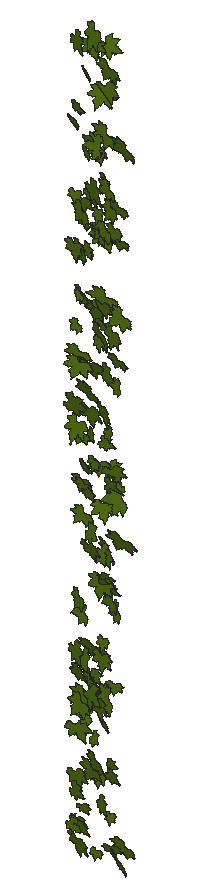
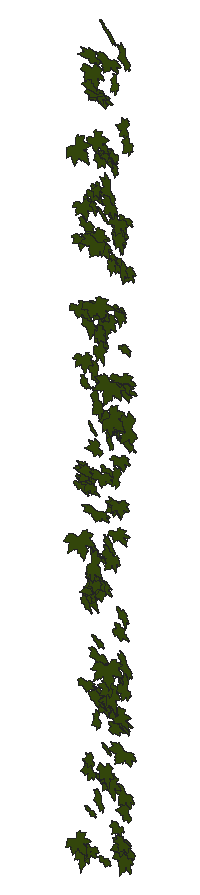
# SketchUp Ruby script. Lengths in inches.
U = 1.inch
M = Sketchup.active_model
def pt(a) = Geom::Point3d.new(a.map { |v| v * U })
def face(e, loops, mat)
  f = e.add_face(loops[0].map { |a| pt(a) })
  loops[1..].each { |l| e.add_face(l.map { |a| pt(a) }).erase! }
  f.material = f.back_material = mat if mat
  f
end
# faces: each face lists its corners as indices into pts; further lists are holes
def faces(e, pts, list, mat = nil) = list.each { |f| face(e, (f[0].is_a?(Array) ? f : [f]).map { |l| l.map { |i| pts[i] } }, mat) }
# xy, xz, yz: faces in a plane at the given z, y or x. An outline is a flat list of corners, or four numbers for a rectangle; further outlines are holes
def ring(l) = l.size == 4 ? [[l[0], l[1]], [l[2], l[1]], [l[2], l[3]], [l[0], l[3]]] : l.each_slice(2).to_a
def flat(e, list, mat, &to3) = list.each { |f| face(e, (f[0].is_a?(Array) ? f : [f]).map { |l| ring(l).map { |u, v| to3.(u, v) } }, mat) }
def xy(e, z, list, mat = nil) = flat(e, list, mat) { |x, y| [x, y, z] }
def xz(e, y, list, mat = nil) = flat(e, list, mat) { |x, z| [x, y, z] }
def yz(e, x, list, mat = nil) = flat(e, list, mat) { |y, z| [x, y, z] }
def lines(e, pts, list) = list.each { |a, b| e.add_line(pt(pts[a]), pt(pts[b])) }
# prism: a flat outline (further loops are holes) pulled along v
def prism(e, loops, v, mat = nil)
  f = face(e, loops, mat); d = Geom::Vector3d.new(v.map { |x| x * U })
  f.pushpull(f.normal.samedirection?(d) ? d.length : -d.length)
end
def box(e, o, s, mat = nil) = prism(e, [[o, [o[0] + s[0], o[1], o[2]], [o[0] + s[0], o[1] + s[1], o[2]], [o[0], o[1] + s[1], o[2]]]], [0, 0, s[2]], mat)
def at(x, y, z, deg = 0) = Geom::Transformation.translation(pt([x, y, z])) * Geom::Transformation.rotation(ORIGIN, Z_AXIS, deg.degrees)
def axes(o, x, y, z) = Geom::Transformation.new([*x, 0, *y, 0, *z, 0, *pt(o).to_a, 1])
def part(name) = M.definitions.add(name)
# library, detail: a bought-in or finely detailed component or shape, given as its bounding box
def library(name, o, s) = part(name).tap { |d| box(d.entities, o, s) }
def detail(e, o, s) = box(e.add_group.entities, o, s)
def put(e, d, t, mat = nil) = e.add_instance(d, t).tap { |i| i.material = mat if mat }
def group(e, t, mat = nil) = e.add_group.tap { |g| g.transformation = t; g.material = mat if mat }.entities
root = M.entities
M.materials.add("[Vegetation Blur 03]").color = [83, 114, 18]
c1 = part("ivy")
xy(c1.entities,0,[[0.782,0,0.786,0,0.787,0.005,0.789,0.009,0.821,0.072,0.875,0.147,1.001,0.272,1.073,0.331,1.137,0.363,1.178,0.379,1.223,0.384,1.272,0.383,1.311,0.374,1.36,0.355,1.399,0.334,1.491,0.285,1.541,0.244,1.583,0.199,1.617,0.15,1.64,0.128,1.662,0.115,1.717,0.105,1.745,0.093,1.784,0.054,1.819,0.057,1.854,0.064,1.882,0.075,1.896,0.074,1.91,0.071,1.937,0.063,1.964,0.053,1.99,0.038,2.016,0.015,2.034,0.002,2.04,0,2.038,0.003,2.036,0.007,2.033,0.038,2.036,0.068,2.045,0.1,2.055,0.116,2.064,0.123,2.077,0.129,2.088,0.129,2.106,0.132,2.118,0.13,2.179,0.132,2.207,0.133,2.225,0.133,2.242,0.138,2.22,0.162,2.207,0.186,2.206,0.213,2.212,0.236,2.228,0.262,2.247,0.274,2.298,0.283,2.355,0.294,2.37,0.296,2.376,0.295,2.377,0.3,2.377,0.303,2.385,0.329,2.411,0.37,2.426,0.392,2.449,0.407,2.511,0.426,2.561,0.444,2.619,0.466,2.589,0.469,2.561,0.476,2.501,0.5,2.449,0.516,2.424,0.523,2.401,0.535,2.377,0.556,2.372,0.568,2.36,0.575,2.268,0.586,2.225,0.592,2.207,0.599,2.194,0.61,2.143,0.65,2.13,0.664,2.122,0.682,2.123,0.7,2.13,0.719,2.148,0.75,2.17,0.781,2.195,0.807,2.221,0.828,2.284,0.874,2.291,0.88,2.288,0.887,2.276,0.9,2.267,0.916,2.265,0.933,2.273,0.967,2.292,1.002,2.313,1.03,2.334,1.054,2.348,1.067,2.358,1.074,2.363,1.076,2.362,1.081,2.35,1.094,2.347,1.11,2.35,1.143,2.359,1.18,2.385,1.254,2.415,1.324,2.448,1.393,2.45,1.4,2.446,1.398,2.44,1.394,2.427,1.383,2.402,1.36,2.376,1.339,2.345,1.324,2.305,1.309,2.282,1.303,2.273,1.306,2.245,1.294,2.212,1.287,2.187,1.291,2.163,1.301,2.142,1.316,2.134,1.327,2.124,1.325,2.09,1.292,2.053,1.259,2.014,1.234,1.973,1.215,1.954,1.21,1.931,1.208,1.909,1.212,1.893,1.22,1.879,1.233,1.872,1.248,1.867,1.281,1.864,1.319,1.821,1.258,1.773,1.197,1.726,1.141,1.698,1.121,1.679,1.116,1.666,1.117,1.647,1.122,1.632,1.129,1.62,1.141,1.617,1.154,1.617,1.219,1.621,1.254,1.623,1.268,1.623,1.281,1.618,1.314,1.606,1.346,1.603,1.375,1.607,1.403,1.603,1.467,1.599,1.499,1.605,1.525,1.614,1.552,1.629,1.577,1.635,1.589,1.629,1.587,1.618,1.582,1.596,1.566,1.581,1.556,1.568,1.552,1.557,1.55,1.545,1.553,1.531,1.562,1.522,1.572,1.504,1.591,1.486,1.611,1.474,1.631,1.457,1.666,1.455,1.684,1.457,1.698,1.452,1.715,1.444,1.728,1.424,1.754,1.419,1.772,1.423,1.786,1.434,1.819,1.444,1.848,1.446,1.855,1.44,1.861,1.43,1.867,1.386,1.904,1.349,1.948,1.326,1.973,1.31,1.995,1.288,2.048,1.284,2.153,1.287,2.254,1.284,2.255,1.282,2.253,1.278,2.247,1.274,2.237,1.266,2.216,1.226,2.125,1.208,2.076,1.184,2.033,1.155,1.984,1.135,1.942,1.111,1.899,1.083,1.861,1.053,1.85,1.059,1.83,1.061,1.809,1.056,1.79,1.049,1.767,1.04,1.749,1.018,1.733,0.994,1.726,0.942,1.734,0.95,1.6875,0.944,1.645,0.932,1.608,0.911,1.585,0.881,1.58,0.854,1.582,0.828,1.588,0.785,1.618,0.773,1.625,0.775,1.614,0.779,1.598,0.796,1.502,0.818,1.402,0.861,1.283,0.882,1.224,0.894,1.174,0.892,1.148,0.886,1.123,0.881,1.107,0.872,1.099,0.849,1.094,0.818,1.092,0.789,1.098,0.762,1.107,0.753,1.113,0.721,1.139,0.698,1.163,0.678,1.194,0.665,1.224,0.628,1.28,0.612,1.312,0.606,1.327,0.606,1.314,0.599,1.282,0.594,1.267,0.581,1.256,0.544,1.245,0.512,1.244,0.473,1.249,0.444,1.256,0.382,1.288,0.339,1.306,0.324,1.316,0.317,1.324,0.309,1.326,0.27,1.314,0.227,1.313,0.185,1.3125,0.152,1.317,0.122,1.328,0.092,1.345,0.073,1.353,0.079,1.338,0.092,1.308,0.117,1.249,0.13,1.215,0.139,1.164,0.147,1.148,0.157,1.136,0.163,1.122,0.174,1.086,0.177,1.067,0.182,1.054,0.186,1.043,0.191,1.038,0.211,1.028,0.237,1.005,0.25,0.974,0.253,0.96,0.25,0.944,0.242,0.914,0.243,0.906,0.249,0.902,0.26,0.894,0.289,0.88,0.307,0.873,0.322,0.862,0.364,0.799,0.403,0.738,0.431,0.709,0.439,0.691,0.441,0.678,0.4375,0.66,0.428,0.645,0.394,0.623,0.303,0.594,0.255,0.581,0.214,0.577,0.179,0.573,0.173,0.568,0.175,0.561,0.167,0.55,0.141,0.523,0.113,0.503,0.077,0.49,0.045,0.486,0.026,0.485,0.019,0.486,0.011,0.483,0,0.471,0.014,0.467,0.044,0.455,0.058,0.447,0.07,0.438,0.097,0.411,0.125,0.394,0.158,0.377,0.174,0.366,0.182,0.359,0.185,0.361,0.242,0.331,0.253,0.316,0.258,0.303,0.262,0.283,0.274,0.278,0.308,0.274,0.341,0.252,0.366,0.226,0.366,0.222,0.37,0.22,0.38,0.221,0.395,0.221,0.425,0.216,0.45,0.207,0.465,0.192,0.473,0.178,0.484,0.15,0.489,0.116,0.483,0.089,0.468,0.058,0.45,0.035,0.435,0.018,0.429,0.011,0.434,0.012,0.438,0.014,0.469,0.019,0.542,0.016,0.581,0.015,0.612,0.027,0.68,0.055,0.696,0.057,0.712,0.052,0.73,0.045,0.741,0.036,0.766,0.014]])
put(root,c1,axes([79.86,173.7,54.72],[0.18512,0.00647,0.33943],[0.41367,-0.0999,-0.14998],[-0.04308,-0.93144,0.01844]),"[Vegetation Blur 03]")
put(root,c1,axes([80.13,173.7,87.79],[0.32765,-0.02489,0.01881],[0.02157,-0.07508,-0.26601],[-0.01455,-0.67173,0.02903]),"[Vegetation Blur 03]")
put(root,c1,axes([80.16,173.7,79.85],[0.50815,0.02983,-0.17456],[-0.21367,-0.02159,-0.41487],[0.01743,-1.13431,0.00331]),"[Vegetation Blur 03]")
put(root,c1,axes([80.49,173.7,81.24],[0.24945,-0.08617,-0.15972],[-0.19859,-0.02674,-0.20432],[-0.02483,-0.6519,0.02949]),"[Vegetation Blur 03]")
put(root,c1,axes([80.01,173.7,91.5625],[0.34754,-0.2147,0.09746],[0.13272,0.06991,-0.29103],[-0.08677,-0.75297,-0.05481]),"[Vegetation Blur 03]")
put(root,c1,axes([81.18,173.7,78.04],[0.15268,0.21133,-0.48982],[-0.60568,0.18355,-0.11329],[-0.06257,-1.26109,-0.09857]),"[Vegetation Blur 03]")
put(root,c1,axes([80.14,173.7,79.3],[0.55742,0.02012,-0.13001],[-0.15728,-0.13301,-0.4524],[0.0271,-1.18554,0.04855]),"[Vegetation Blur 03]")
put(root,c1,axes([79.89,173.7,85.24],[0.58629,-0.17522,0.04019],[0.04988,0.00183,-0.48347],[-0.08478,-1.21072,-0.00655]),"[Vegetation Blur 03]")
put(root,c1,axes([80.37,173.7,75.5],[0.38921,0.02788,-0.11804],[-0.14492,0.01541,-0.31769],[0.01009,-0.85429,-0.00958]),"[Vegetation Blur 03]")
put(root,c1,axes([80.71,173.7,87.32],[0.36249,-0.1648,-0.3565],[-0.41016,0.32061,-0.3011],[-0.17026,-1.12322,-0.03364]),"[Vegetation Blur 03]")
put(root,c1,axes([80.36,173.7,73.16],[0.40951,0.01971,-0.10583],[-0.13003,0.06915,-0.33309],[-0.00105,-0.88123,-0.0285]),"[Vegetation Blur 03]")
put(root,c1,axes([80.13,173.7,55.37],[0.37849,-0.06704,0.09137],[0.11442,0.06293,-0.30843],[-0.02244,-0.80977,-0.03153]),"[Vegetation Blur 03]")
put(root,c1,axes([79.76,173.7,60.03],[0.53376,0.03726,0.21952],[0.269,0.00727,-0.43585],[0.01776,-1.22992,0.00407]),"[Vegetation Blur 03]")
put(root,c1,axes([80.72,173.7,62.45],[0.42826,-0.11256,-0.35023],[-0.42906,0.04831,-0.35189],[-0.05529,-1.24664,0.01798]),"[Vegetation Blur 03]")
put(root,c1,axes([79.82,173.7,76.28],[0.20202,-0.16973,0.51163],[0.63222,0.07532,-0.16235],[0.00985,-1.35325,-0.07321]),"[Vegetation Blur 03]")
put(root,c1,axes([81.05,173.7,66.72],[0.19822,-0.13225,-0.36337],[-0.44645,0.06503,-0.16594],[-0.0552,-1.0008,0.03723]),"[Vegetation Blur 03]")
put(root,c1,axes([80.13,173.7,56.5],[0.13655,-0.05783,0.35944],[0.43753,-0.10617,-0.1134],[-0.05764,-0.9429,-0.00928]),"[Vegetation Blur 03]")
put(root,c1,axes([80.49,173.7,62.03],[0.51915,-0.17766,-0.225],[-0.28069,-0.03421,-0.42714],[-0.06834,-1.20911,0.04515]),"[Vegetation Blur 03]")
put(root,c1,axes([79.91,173.7,57.74],[0.52125,-0.12471,0.19571],[0.23821,-0.0569,-0.42827],[-0.06661,-1.17932,-0.00003]),"[Vegetation Blur 03]")
put(root,c1,axes([80.65,173.7,71.69],[0.40363,-0.02669,-0.22372],[-0.27442,-0.04788,-0.32887],[0.00236,-1.00289,0.02165]),"[Vegetation Blur 03]")
put(root,c1,axes([80.59,173.7,73.06],[0.38167,-0.01698,-0.15187],[-0.18516,0.0606,-0.31101],[-0.02031,-0.87168,-0.01866]),"[Vegetation Blur 03]")
put(root,c1,axes([80.47,173.7,67.37],[0.45232,-0.27078,-0.13351],[-0.16346,0.04761,-0.38403],[-0.13176,-0.98864,0.01808]),"[Vegetation Blur 03]")
put(root,c1,axes([80.62,173.7,82.86],[0.28246,-0.12607,-0.06429],[-0.08477,-0.04633,-0.23378],[-0.05266,-0.60166,0.03147]),"[Vegetation Blur 03]")
put(root,c1,axes([80.58,173.7,87.18],[0.47471,-0.2198,-0.23723],[-0.27334,0.21714,-0.39597],[-0.14555,-1.12467,-0.03009]),"[Vegetation Blur 03]")
put(root,c1,axes([81.07,173.7,79.25],[0.13027,0.06294,-0.24641],[-0.30303,0.06322,-0.10416],[-0.01626,-0.67369,-0.0328]),"[Vegetation Blur 03]")
put(root,c1,axes([80.01,173.7,54.72],[0.66178,-0.29714,0.00728],[0.02239,0.12543,-0.55031],[-0.14293,-1.35615,-0.0525]),"[Vegetation Blur 03]")
put(root,c1,axes([80.57,173.7,87.5],[0.50423,-0.25138,-0.23976],[-0.28758,0.12452,-0.42338],[-0.1361,-1.1944,0.00632]),"[Vegetation Blur 03]")
put(root,c1,axes([80.39,173.7,91.92],[0.06833,-0.14193,0.31087],[0.38368,-0.0807,-0.06197],[-0.05132,-0.79223,-0.04938]),"[Vegetation Blur 03]")
put(root,c1,axes([80.48,173.7,85.44],[0.499,-0.30069,-0.16614],[-0.19194,0.14146,-0.42426],[-0.16109,-1.09995,-0.00914]),"[Vegetation Blur 03]")
put(root,c1,axes([80.16,173.7,76.24],[0.61381,-0.2023,0.00115],[-0.01893,-0.26118,-0.49641],[-0.09648,-1.23581,0.10472]),"[Vegetation Blur 03]")
put(root,c1,axes([80.52,173.7,83.02],[0.4623,-0.23108,-0.11744],[-0.13279,0.12742,-0.38762],[-0.12523,-0.98816,-0.02252]),"[Vegetation Blur 03]")
put(root,c1,axes([80.3,173.7,87.6],[0.49002,-0.06773,0.03255],[0.04203,0.06603,-0.39982],[-0.03013,-1.00954,-0.02833]),"[Vegetation Blur 03]")
put(root,c1,axes([80.17,173.7,62.87],[0.2552,-0.21443,0.36363],[0.45118,-0.05704,-0.2162],[-0.07626,-1.05507,-0.06222]),"[Vegetation Blur 03]")
put(root,c1,axes([80.04,173.7,64.1],[0.40591,-0.18014,0.3374],[0.39655,-0.24525,-0.33836],[-0.14603,-1.16675,0.01903]),"[Vegetation Blur 03]")
put(root,c1,axes([80.51,173.7,56.02],[0.2717,-0.01326,0.11926],[0.14597,0.06528,-0.22036],[0.00938,-0.63148,-0.02528]),"[Vegetation Blur 03]")
put(root,c1,axes([80.29,173.7,54.9],[0.29257,-0.13243,0.26003],[0.3239,0.04481,-0.23915],[-0.02726,-0.88901,-0.05079]),"[Vegetation Blur 03]")
put(root,c1,axes([80.16,173.7,95.55],[0.32606,-0.15993,0.37004],[0.43652,-0.25327,-0.27342],[-0.14515,-1.12098,0.00898]),"[Vegetation Blur 03]")
put(root,c1,axes([81.08,173.7,63.5625],[0.44681,-0.13861,-0.40686],[-0.47518,0.33403,-0.36549],[-0.1651,-1.33648,-0.04915]),"[Vegetation Blur 03]")
put(root,c1,axes([81.5,173.7,61.41],[0.05855,-0.11186,-0.32035],[-0.39567,-0.06136,-0.0448],[0.02177,-0.81436,0.04738]),"[Vegetation Blur 03]")
put(root,c1,axes([80.75,173.7,64.84],[0.5883,0.12569,-0.22776],[-0.28567,0.25569,-0.4693],[0.00068,-1.31528,-0.113]),"[Vegetation Blur 03]")
put(root,c1,axes([80.97,173.7,90.33],[0.2858,-0.16556,-0.09391],[-0.1058,0.0991,-0.24194],[-0.0923,-0.62621,-0.01346]),"[Vegetation Blur 03]")
put(root,c1,axes([80.41,173.7,79.23],[0.67545,-0.01499,0.0047],[0.00705,0.26519,-0.54115],[-0.00605,-1.36446,-0.10523]),"[Vegetation Blur 03]")
put(root,c1,axes([81.05,173.7,85.39],[0.30779,-0.16022,-0.12096],[-0.12595,0.19898,-0.2549],[-0.11031,-0.67423,-0.04648]),"[Vegetation Blur 03]")
put(root,c1,axes([80.5625,173.7,63.51],[0.22572,0.02556,0.3673],[0.42622,-0.34586,-0.17068],[-0.14503,-0.97663,0.07006]),"[Vegetation Blur 03]")
put(root,c1,axes([80.84,173.7,90.75],[0.27595,-0.07999,0.10883],[0.13684,0.05207,-0.2251],[-0.02378,-0.62852,-0.0325]),"[Vegetation Blur 03]")
put(root,c1,axes([81,173.7,58.78],[0.5571,-0.15804,-0.2532],[-0.30286,0.14883,-0.45846],[-0.10211,-1.30372,-0.02164]),"[Vegetation Blur 03]")
put(root,c1,axes([80.73,173.7,84.92],[0.26922,-0.1042,0.25304],[0.30661,-0.09593,-0.2235],[-0.06845,-0.83952,-0.00587]),"[Vegetation Blur 03]")
put(root,c1,axes([80.91,173.7,73.57],[0.07402,-0.1812,0.31745],[0.39109,-0.12634,-0.07209],[-0.07805,-0.80492,-0.06015]),"[Vegetation Blur 03]")
put(root,c1,axes([80.85,173.7,94.38],[0.3403,-0.29163,0.09942],[0.13762,0.03874,-0.29588],[-0.12643,-0.74278,-0.05447]),"[Vegetation Blur 03]")
put(root,c1,axes([80.82,173.7,72.4],[0.28875,-0.1223,0.18363],[0.229,0.01809,-0.23796],[-0.04139,-0.75306,-0.03554]),"[Vegetation Blur 03]")
put(root,c1,axes([80.6,173.7,76.96],[0.63148,-0.16792,0.0994],[0.12538,0.04433,-0.51879],[-0.07597,-1.32267,-0.03001]),"[Vegetation Blur 03]")
put(root,c1,axes([80.86,173.7,62.93],[0.31712,0.01449,0.22059],[0.2693,0.0595,-0.25849],[0.0241,-0.85537,-0.01424]),"[Vegetation Blur 03]")
put(root,c1,axes([80.71,173.7,95.6875],[0.52799,0.03971,0.1403],[0.17249,-0.03446,-0.43082],[0.01316,-1.14211,0.01788]),"[Vegetation Blur 03]")
put(root,c1,axes([81,173.7,82.47],[0.55471,-0.15442,-0.09413],[-0.10485,0.16405,-0.45388],[-0.08911,-1.1543,-0.05191]),"[Vegetation Blur 03]")
put(root,c1,axes([80.72,173.7,69.86],[0.52924,-0.21641,0.13482],[0.17446,0.07604,-0.43695],[-0.08896,-1.13835,-0.05482]),"[Vegetation Blur 03]")
put(root,c1,axes([81.3125,173.7,59.23],[0.48731,-0.17978,-0.24983],[-0.29064,0.21865,-0.40235],[-0.12987,-1.16387,-0.037]),"[Vegetation Blur 03]")
put(root,c1,axes([81.03,173.7,70.02],[0.07963,0.08394,0.36792],[0.43963,-0.2386,-0.05481],[-0.10777,-0.91131,0.04824]),"[Vegetation Blur 03]")
put(root,c1,axes([81.71,173.7,86.43],[0.27575,-0.07071,-0.32237],[-0.38727,0.16418,-0.22631],[-0.08498,-0.9776,-0.01469]),"[Vegetation Blur 03]")
put(root,c1,axes([81.58,173.7,90.93],[0.3287,-0.1611,-0.24597],[-0.30329,0.03864,-0.27395],[-0.07054,-0.91688,0.03167]),"[Vegetation Blur 03]")
put(root,c1,axes([80.88,173.7,87.98],[0.42324,-0.15513,0.17492],[0.21736,0.00516,-0.3496],[-0.06611,-0.97622,-0.02964]),"[Vegetation Blur 03]")
put(root,c1,axes([82.03,173.7,91.27],[0.20332,-0.17652,-0.4378],[-0.54125,0.03497,-0.16965],[-0.04646,-1.17997,0.06046]),"[Vegetation Blur 03]")
put(root,c1,axes([81.26,173.7,62.13],[0.08923,-0.0651,0.22881],[0.28147,0.0622,-0.07033],[0.01942,-0.60224,-0.032]),"[Vegetation Blur 03]")
put(root,c1,axes([81.3,173.7,74.42],[0.35274,-0.11868,-0.02991],[-0.03922,-0.02703,-0.29129],[-0.05595,-0.72928,0.01566]),"[Vegetation Blur 03]")
put(root,c1,axes([81.29,173.7,59.58],[0.08406,0.07505,0.23958],[0.28752,-0.16835,-0.0589],[-0.06954,-0.60538,0.04608]),"[Vegetation Blur 03]")
put(root,c1,axes([81.18,173.7,75.51],[0.18332,-0.13201,0.23981],[0.28131,-0.17522,-0.15841],[-0.10639,-0.6908,-0.00565]),"[Vegetation Blur 03]")
put(root,c1,axes([82.29,173.7,70.12],[0.10735,0.13666,-0.49936],[-0.59338,0.3622,-0.06937],[-0.16335,-1.22594,-0.07616]),"[Vegetation Blur 03]")
put(root,c1,axes([81.4,173.7,54.17],[0.29298,-0.03076,-0.00517],[-0.00747,-0.046,-0.2387],[-0.01442,-0.60127,0.01853]),"[Vegetation Blur 03]")
put(root,c1,axes([81.86,173.7,81.08],[0.29122,-0.09132,-0.34949],[-0.40801,0.28097,-0.238],[-0.13739,-1.02797,-0.034]),"[Vegetation Blur 03]")
put(root,c1,axes([82,173.7,81.86],[0.15958,-0.02123,-0.31626],[-0.37905,0.17205,-0.12921],[-0.08118,-0.84504,-0.01836]),"[Vegetation Blur 03]")
put(root,c1,axes([80.88,173.7,61.62],[0.16056,0.04012,0.53459],[0.63688,-0.33645,-0.12344],[-0.15436,-1.34643,0.04677]),"[Vegetation Blur 03]")
put(root,c1,axes([81.23,173.7,74.21],[0.45127,0.0715,0.00789],[0.01018,-0.0128,-0.36935],[0.0346,-0.92876,0.0057]),"[Vegetation Blur 03]")
put(root,c1,axes([81.72,173.7,83.38],[0.53259,0.07407,-0.33493],[-0.4092,-0.06459,-0.43565],[0.04766,-1.38209,0.00241]),"[Vegetation Blur 03]")
put(root,c1,axes([82.09,173.7,91.9375],[0.36403,-0.06267,-0.40957],[-0.5016,0.04126,-0.29795],[-0.03412,-1.27511,0.01049]),"[Vegetation Blur 03]")
put(root,c1,axes([82.07,173.7,89.21],[0.19632,-0.0358,-0.23719],[-0.2774,0.19596,-0.15758],[-0.08838,-0.69459,-0.03223]),"[Vegetation Blur 03]")
put(root,c1,axes([81.58,173.7,90.38],[0.31483,-0.06922,0.03461],[0.04453,0.03834,-0.25772],[-0.03078,-0.65259,-0.01881]),"[Vegetation Blur 03]")
put(root,c1,axes([81.85,173.7,86.875],[0.46325,-0.03451,-0.29794],[-0.36488,0.02419,-0.37832],[-0.02045,-1.21347,0.00093]),"[Vegetation Blur 03]")
put(root,c1,axes([81.33,173.7,97],[0.61554,-0.40401,-0.01131],[-0.04771,-0.21545,-0.519],[-0.19095,-1.24853,0.09322]),"[Vegetation Blur 03]")
put(root,c1,axes([81.55,173.7,81.5],[0.58606,-0.32249,-0.17371],[-0.19607,0.18401,-0.49434],[-0.17725,-1.2698,-0.02752]),"[Vegetation Blur 03]")
put(root,c1,axes([80.99,173.7,88.22],[0.41734,-0.25524,0.42347],[0.50918,-0.21404,-0.35453],[-0.15923,-1.35344,-0.02379]),"[Vegetation Blur 03]")
put(root,c1,axes([81.62,173.7,58.16],[0.34421,-0.10508,0.04416],[0.04441,-0.1326,-0.28022],[-0.05969,-0.70465,0.04615]),"[Vegetation Blur 03]")
put(root,c1,axes([81.58,173.7,87.36],[0.35292,-0.17211,0.08002],[0.07901,-0.17569,-0.29156],[-0.10181,-0.73298,0.0511]),"[Vegetation Blur 03]")
put(root,c1,axes([81.55,173.7,80.67],[0.3385,-0.12078,0.12895],[0.14584,-0.15588,-0.27795],[-0.08451,-0.75275,0.03687]),"[Vegetation Blur 03]")
put(root,c1,axes([81.34,173.7,68.47],[0.64834,-0.11558,0.00243],[-0.00125,-0.10055,-0.52962],[-0.05623,-1.33037,0.03982]),"[Vegetation Blur 03]")
put(root,c1,axes([82.33,173.7,89.03],[0.26205,-0.06963,-0.34462],[-0.42004,0.08964,-0.2156],[-0.05487,-1.01871,0.00458]),"[Vegetation Blur 03]")
put(root,c1,axes([81.55,173.7,93.82],[0.58164,-0.02914,-0.08506],[-0.10504,-0.22356,-0.46637],[0.00547,-1.19524,0.0893]),"[Vegetation Blur 03]")
put(root,c1,axes([82.47,173.7,63.02],[0.29249,-0.26424,-0.46367],[-0.56799,0.1604,-0.25303],[-0.12902,-1.30512,0.06278]),"[Vegetation Blur 03]")
put(root,c1,axes([81.86,173.7,68.43],[0.29824,-0.02143,-0.02343],[-0.02665,0.10046,-0.24043],[-0.01491,-0.60833,-0.03888]),"[Vegetation Blur 03]")
put(root,c1,axes([81.21,173.7,86.03],[0.60611,0.08882,0.16972],[0.20851,-0.00255,-0.49577],[0.04043,-1.31863,0.01239]),"[Vegetation Blur 03]")
put(root,c1,axes([81.375,173.7,72.07],[0.5345,0.11261,0.12686],[0.16236,-0.17388,-0.43135],[0.02823,-1.13219,0.07887]),"[Vegetation Blur 03]")
put(root,c1,axes([81.55,173.7,82.49],[0.44672,-0.11391,0.09884],[0.12385,0.0351,-0.3665],[-0.0489,-0.9518,-0.02535]),"[Vegetation Blur 03]")
put(root,c1,axes([81.8125,173.7,65.28],[0.33589,-0.10606,0.03492],[0.03467,-0.10992,-0.27466],[-0.05731,-0.68805,0.03849]),"[Vegetation Blur 03]")
put(root,c1,axes([81.28,173.7,62.03],[0.57796,-0.29472,0.19025],[0.2281,-0.10009,-0.48593],[-0.15109,-1.27852,-0.00582]),"[Vegetation Blur 03]")
put(root,c1,axes([81.71,173.7,90.2],[0.24496,-0.07431,0.21292],[0.23492,-0.26987,-0.19483],[-0.11909,-0.6852,0.05364]),"[Vegetation Blur 03]")
put(root,c1,axes([81.5,173.7,64.54],[0.56428,-0.16916,0.04285],[0.04868,-0.06133,-0.46503],[-0.08453,-1.16458,0.01826]),"[Vegetation Blur 03]")
put(root,c1,axes([81.55,173.7,69.47],[0.29882,0.02623,0.28715],[0.33985,-0.26962,-0.23169],[-0.09199,-0.91085,0.07685]),"[Vegetation Blur 03]")
put(root,c1,axes([81.77,173.7,74.99],[0.12471,-0.00455,0.29508],[0.36083,0.05141,-0.10146],[0.0229,-0.78534,-0.00835]),"[Vegetation Blur 03]")
put(root,c1,axes([81.93,173.7,95.26],[0.56003,-0.11483,-0.22477],[-0.26984,0.13286,-0.4585],[-0.07841,-1.27735,-0.02748]),"[Vegetation Blur 03]")
put(root,c1,axes([81.5625,173.7,68.17],[0.35675,-0.1356,0.28151],[0.35114,0.1247,-0.28695],[-0.00453,-1.0135,-0.07297]),"[Vegetation Blur 03]")
put(root,c1,axes([82.49,173.7,67.94],[0.31943,-0.14813,-0.35105],[-0.42397,0.15166,-0.26703],[-0.10221,-1.09204,0.01053]),"[Vegetation Blur 03]")
put(root,c1,axes([81.69,173.7,56.52],[0.23742,-0.1267,0.33587],[0.39552,-0.23419,-0.20013],[-0.12927,-0.94922,0.00454]),"[Vegetation Blur 03]")
put(root,c1,axes([81.8125,173.7,95.25],[0.0857,0.17777,0.39101],[0.48593,0.02942,-0.07304],[0.02949,-1.0011,0.06729]),"[Vegetation Blur 03]")
put(root,c1,axes([81.9,173.7,60.93],[0.26661,-0.22568,0.1584],[0.20153,-0.02212,-0.2309],[-0.09528,-0.67823,-0.04518]),"[Vegetation Blur 03]")
put(root,c1,axes([81.58,173.7,67.58],[0.27593,-0.17427,0.39331],[0.48854,0.16147,-0.21704],[0.02723,-1.13128,-0.09157]),"[Vegetation Blur 03]")
put(root,c1,axes([81.99,173.7,54.52],[0.36983,0.02306,0.04655],[0.05424,0.13467,-0.29755],[0.02088,-0.75816,-0.05144]),"[Vegetation Blur 03]")
put(root,c1,axes([81.51,173.7,93.69],[0.56787,-0.08069,0.24242],[0.2938,-0.10677,-0.464],[-0.05873,-1.31444,0.02281]),"[Vegetation Blur 03]")
put(root,c1,axes([82.03,173.7,78.59],[0.06006,-0.04189,0.40073],[0.47866,-0.22553,-0.0515],[-0.11129,-0.99263,-0.00521]),"[Vegetation Blur 03]")
put(root,c1,axes([81.93,173.7,69.59],[0.33061,-0.13828,0.23143],[0.27228,-0.16795,-0.27487],[-0.10387,-0.88042,0.01609]),"[Vegetation Blur 03]")
put(root,c1,axes([82.15,173.7,75.97],[0.2323,-0.07315,0.16912],[0.19295,-0.17827,-0.18866],[-0.08352,-0.61528,0.03456]),"[Vegetation Blur 03]")
put(root,c1,axes([81.72,173.7,77.38],[0.56286,-0.41503,0.17137],[0.21267,-0.05627,-0.48669],[-0.19885,-1.23496,-0.03542]),"[Vegetation Blur 03]")
put(root,c1,axes([82.26,173.7,56.3],[0.28663,-0.07213,0.05383],[0.05877,-0.11436,-0.23255],[-0.04609,-0.59433,0.03821]),"[Vegetation Blur 03]")
put(root,c1,axes([82.32,173.7,88.08],[0.46163,-0.2581,-0.13642],[-0.17424,-0.01487,-0.3883],[-0.11538,-1.01019,0.04057]),"[Vegetation Blur 03]")
put(root,c1,axes([82.2,173.7,73.63],[0.07333,0.12212,0.31359],[0.38829,0.01811,-0.06159],[0.01986,-0.80476,0.0462]),"[Vegetation Blur 03]")
put(root,c1,axes([82.3,173.7,58.65],[0.09053,-0.05831,0.23092],[0.28382,-0.01925,-0.07488],[-0.01758,-0.61103,-0.01968]),"[Vegetation Blur 03]")
put(root,c1,axes([82.28,173.7,63.08],[0.35798,0.03491,0.00358],[0.00487,-0.0205,-0.29237],[0.01684,-0.73641,0.00831]),"[Vegetation Blur 03]")
put(root,c1,axes([82.47,173.7,80.12],[0.41941,-0.00434,-0.1684],[-0.2031,0.16133,-0.33757],[-0.03648,-0.94822,-0.05667]),"[Vegetation Blur 03]")
put(root,c1,axes([81.875,173.7,73.9],[0.48195,0.00963,0.21143],[0.25864,0.04977,-0.39304],[0.01557,-1.12486,-0.01558]),"[Vegetation Blur 03]")
put(root,c1,axes([82.5625,173.7,88.09],[0.40291,0.01111,-0.21009],[-0.25613,0.11786,-0.3262],[-0.02632,-0.9768,-0.04175]),"[Vegetation Blur 03]")
put(root,c1,axes([83.08,173.7,78.88],[0.08976,-0.09939,-0.28739],[-0.34963,0.10974,-0.07871],[-0.06393,-0.7397,0.02694]),"[Vegetation Blur 03]")
put(root,c1,axes([83.09,173.7,91.4],[0.2991,0.11532,-0.48246],[-0.59082,0.19391,-0.23668],[-0.05934,-1.34945,-0.07524]),"[Vegetation Blur 03]")
put(root,c1,axes([82.46,173.7,70.99],[0.56725,0.10726,-0.27566],[-0.34171,0.20149,-0.45603],[-0.00596,-1.34353,-0.0904]),"[Vegetation Blur 03]")
put(root,c1,axes([82.92,173.7,67.48],[0.25494,-0.21897,-0.29058],[-0.35433,0.12452,-0.22182],[-0.11199,-0.89248,0.04035]),"[Vegetation Blur 03]")
put(root,c1,axes([82.16,173.7,58.08],[0.21568,-0.13397,0.30172],[0.37321,-0.01782,-0.17894],[-0.04036,-0.88058,-0.04228]),"[Vegetation Blur 03]")
put(root,c1,axes([82.34,173.7,86.82],[0.45457,-0.14322,-0.01986],[-0.02603,-0.01905,-0.37516],[-0.06898,-0.93657,0.01067]),"[Vegetation Blur 03]")
put(root,c1,axes([82.97,173.7,55.27],[0.36107,0.086,-0.36328],[-0.44668,0.11955,-0.29126],[-0.01905,-1.17336,-0.0563]),"[Vegetation Blur 03]")
put(root,c1,axes([82.21,173.7,72.8],[0.10325,-0.14377,0.42811],[0.52829,-0.03594,-0.08677],[-0.03077,-1.09956,-0.05314]),"[Vegetation Blur 03]")
put(root,c1,axes([82.26,173.7,81.7],[0.59158,-0.31026,-0.0564],[-0.07139,-0.00087,-0.49803],[-0.1497,-1.22563,0.01463]),"[Vegetation Blur 03]")
put(root,c1,axes([82.5,173.7,54.52],[0.54071,-0.2448,-0.19934],[-0.20803,0.34691,-0.44288],[-0.17473,-1.17061,-0.08956]),"[Vegetation Blur 03]")
put(root,c1,axes([83.26,173.7,73.6875],[0.30037,-0.23448,-0.48095],[-0.59958,-0.05449,-0.24524],[-0.02777,-1.36002,0.09275]),"[Vegetation Blur 03]")
put(root,c1,axes([82.57,173.7,86.13],[0.37713,0.02521,-0.05482],[-0.06814,0.09104,-0.30568],[0.00422,-0.78299,-0.03731]),"[Vegetation Blur 03]")
put(root,c1,axes([82.875,173.7,82.76],[0.44525,-0.05596,-0.30949],[-0.38019,-0.06333,-0.36251],[-0.0007,-1.20185,0.03351]),"[Vegetation Blur 03]")
